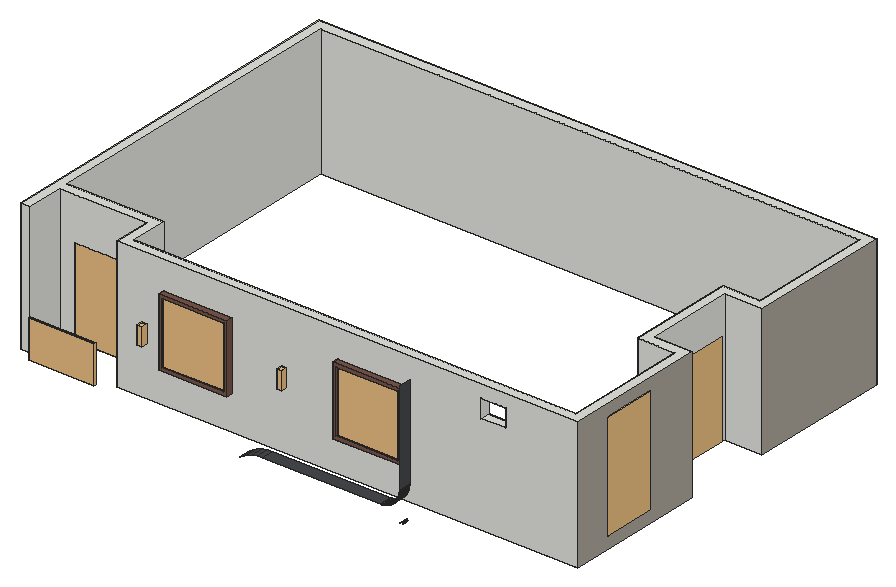
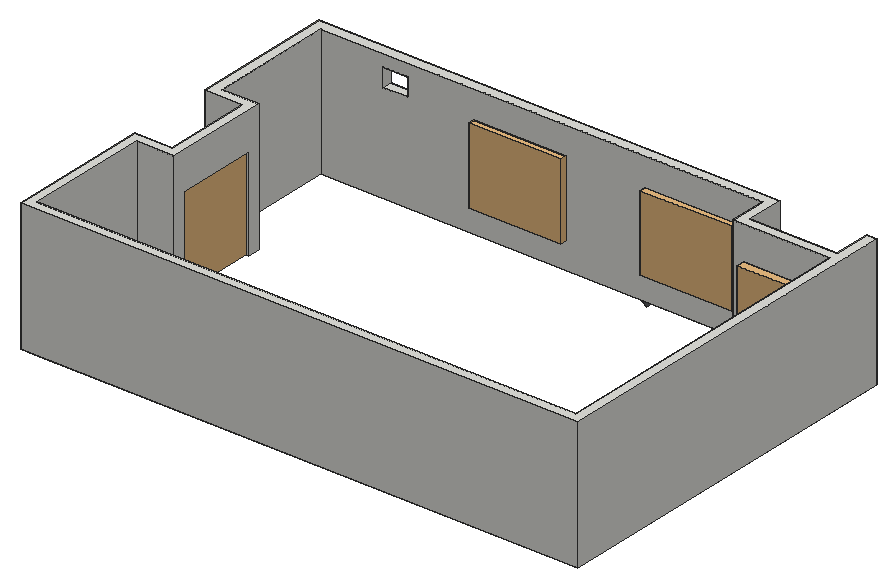
# SketchUp Ruby script. Lengths in inches.
U = 1.inch
M = Sketchup.active_model
def pt(a) = Geom::Point3d.new(a.map { |v| v * U })
def face(e, loops, mat)
  f = e.add_face(loops[0].map { |a| pt(a) })
  loops[1..].each { |l| e.add_face(l.map { |a| pt(a) }).erase! }
  f.material = f.back_material = mat if mat
  f
end
# faces: each face lists its corners as indices into pts; further lists are holes
def faces(e, pts, list, mat = nil) = list.each { |f| face(e, (f[0].is_a?(Array) ? f : [f]).map { |l| l.map { |i| pts[i] } }, mat) }
# xy, xz, yz: faces in a plane at the given z, y or x. An outline is a flat list of corners, or four numbers for a rectangle; further outlines are holes
def ring(l) = l.size == 4 ? [[l[0], l[1]], [l[2], l[1]], [l[2], l[3]], [l[0], l[3]]] : l.each_slice(2).to_a
def flat(e, list, mat, &to3) = list.each { |f| face(e, (f[0].is_a?(Array) ? f : [f]).map { |l| ring(l).map { |u, v| to3.(u, v) } }, mat) }
def xy(e, z, list, mat = nil) = flat(e, list, mat) { |x, y| [x, y, z] }
def xz(e, y, list, mat = nil) = flat(e, list, mat) { |x, z| [x, y, z] }
def yz(e, x, list, mat = nil) = flat(e, list, mat) { |y, z| [x, y, z] }
def lines(e, pts, list) = list.each { |a, b| e.add_line(pt(pts[a]), pt(pts[b])) }
# prism: a flat outline (further loops are holes) pulled along v
def prism(e, loops, v, mat = nil)
  f = face(e, loops, mat); d = Geom::Vector3d.new(v.map { |x| x * U })
  f.pushpull(f.normal.samedirection?(d) ? d.length : -d.length)
end
def box(e, o, s, mat = nil) = prism(e, [[o, [o[0] + s[0], o[1], o[2]], [o[0] + s[0], o[1] + s[1], o[2]], [o[0], o[1] + s[1], o[2]]]], [0, 0, s[2]], mat)
def at(x, y, z, deg = 0) = Geom::Transformation.translation(pt([x, y, z])) * Geom::Transformation.rotation(ORIGIN, Z_AXIS, deg.degrees)
def axes(o, x, y, z) = Geom::Transformation.new([*x, 0, *y, 0, *z, 0, *pt(o).to_a, 1])
def part(name) = M.definitions.add(name)
# library, detail: a bought-in or finely detailed component or shape, given as its bounding box
def library(name, o, s) = part(name).tap { |d| box(d.entities, o, s) }
def detail(e, o, s) = box(e.add_group.entities, o, s)
def put(e, d, t, mat = nil) = e.add_instance(d, t).tap { |i| i.material = mat if mat }
def group(e, t, mat = nil) = e.add_group.tap { |g| g.transformation = t; g.material = mat if mat }.entities
root = M.entities
M.materials.add("1111 AP 9939 Brown seed-N").color = [120, 84, 73]
M.materials.add("1432 AP 8245 TAR ROAD").color = [71, 72, 75]
M.materials.add("Generic").color = [172, 166, 153]
M.materials.add("Outer Light").color = [251, 217, 152]
M.materials.add("[Granite Dark Gray]").color = [69, 68, 68]
M.materials.add("[Wood Cherry Original]").color = [152, 86, 42]
M.materials.add("[Wood Veneer 01]").color = [120, 70, 37]
c1 = library("Group\#43",[0,-2,0],[63,2,36])
c2 = library("WALL LIGHT 69",[4.19,4.05,-8.78],[4.61,5.7,17.13])
c3 = library("Double-hung window 69 in. x 58 in. triple row with mullions",[0,0,-3.59],[62,58,4.59])
c4 = library("Glass Door",[0,0,0],[72,3.54,96])
c5 = library("RIDEAUX \#16",[0,0,0],[103.86,7.74,93.57])
c6 = library("Curtain",[0,0,0],[121.12,7.86,100.24])
c7 = library("SLIDING+GLASS+DOOR",[0,-0.75,0],[72,5.75,80])
c8 = library("Group\#20",[0,0,0],[0.5,51,102])
xy(root,302.79,[[279,95.37,393,107.37],[393,95.37,393.24,107.37]],"1432 AP 8245 TAR ROAD")
yz(root,410.99,[[95.37,320.09,107.37,320.32]],"1432 AP 8245 TAR ROAD")
yz(root,411,[[95.37,320.56,107.37,320.79],[95.37,320.79,107.37,410.79]],"1432 AP 8245 TAR ROAD")
p = [[413.94,96.87,292.75],[414.31,96.87,293.02],[414.31,95.37,293.02],[413.94,95.37,292.75],[411.97,95.37,293.18],[411.61,95.37,292.9375],
  [411.61,96.87,292.9375],[411.97,96.87,293.18],[411.97,96.87,293.18],[411.61,96.87,292.9375],[411.61,95.37,292.9375],[411.97,95.37,293.18],
  [414.67,96.87,293.31],[414.67,95.37,293.31],[414.31,95.37,293.02],[414.67,95.37,293.31],[414.67,96.87,293.31],[414.31,96.87,293.02],
  [412.33,95.37,293.43],[412.33,96.87,293.43],[412.33,96.87,293.43],[412.33,95.37,293.43],[415.03,96.87,293.59],[415.03,95.37,293.59],
  [415.03,95.37,293.59],[415.03,96.87,293.59],[412.69,95.37,293.69],[412.69,96.87,293.69],[412.69,96.87,293.69],[412.69,95.37,293.69],
  [415.38,96.87,293.88],[415.38,95.37,293.88],[415.38,95.37,293.88],[415.38,96.87,293.88],[413.04,95.37,293.95],[413.04,96.87,293.95],
  [413.04,96.87,293.95],[413.04,95.37,293.95],[415.73,96.87,294.18],[415.73,95.37,294.18],[415.73,95.37,294.18],[415.73,96.87,294.18],
  [413.39,95.37,294.21],[413.39,96.87,294.21],[413.39,96.87,294.21],[413.39,95.37,294.21],[413.74,95.37,294.48],[413.74,96.87,294.48],
  [413.74,96.87,294.48],[413.74,95.37,294.48],[416.08,96.87,294.48],[416.08,95.37,294.48],[416.08,95.37,294.48],[416.08,96.87,294.48],
  [414.08,95.37,294.76],[414.08,96.87,294.76],[414.08,96.87,294.76],[414.08,95.37,294.76],[416.42,96.87,294.78],[416.42,95.37,294.78],
  [416.42,95.37,294.78],[416.42,96.87,294.78],[414.42,95.37,295.04],[414.42,96.87,295.04],[414.42,96.87,295.04],[414.42,95.37,295.04],
  [416.76,96.87,295.09],[416.76,95.37,295.09],[416.76,95.37,295.09],[416.76,96.87,295.09],[414.76,95.37,295.32],[414.76,96.87,295.32],
  [414.76,96.87,295.32],[414.76,95.37,295.32],[417.09,96.87,295.4],[417.09,95.37,295.4],[417.09,95.37,295.4],[417.09,96.87,295.4],
  [415.09,95.37,295.61],[415.09,96.87,295.61],[415.09,96.87,295.61],[415.09,95.37,295.61],[261,107.37,297.97],[257.08,107.37,295.35],
  [257.08,95.37,295.35],[261,95.37,297.97],[417.42,96.87,295.72],[417.42,95.37,295.72],[415.42,95.37,295.9],[415.42,96.87,295.9],
  [415.42,96.87,295.9],[415.42,95.37,295.9],[415.74,95.37,296.19],[415.74,96.87,296.19],[415.74,96.87,296.19],[415.74,95.37,296.19],
  [416.06,95.37,296.49],[416.06,96.87,296.49],[416.06,96.87,296.49],[416.06,95.37,296.49],[416.375,95.37,296.8],[416.375,96.87,296.8],
  [416.375,96.87,296.8],[416.375,95.37,296.8],[416.6875,95.37,297.1],[416.6875,96.87,297.1],[416.6875,96.87,297.1],[416.6875,95.37,297.1],
  [417,95.37,297.42],[417,96.87,297.42],[417,96.87,297.42],[417,95.37,297.42],[417.3,95.37,297.73],[417.3,96.87,297.73],
  [417.3,96.87,297.73],[417.3,95.37,297.73],[265.22,107.37,300.05],[265.22,95.37,300.05],[269.68,107.37,301.57],[269.68,95.37,301.57],
  [274.3,107.37,302.48],[274.3,95.37,302.48],[279,107.37,302.79],[279,95.37,302.79],[393.47,107.37,302.8],[393.24,107.37,302.79],
  [393.24,95.37,302.79],[393.47,95.37,302.8],[393.71,107.37,302.81],[393.71,95.37,302.81],[393.94,107.37,302.82],[393.94,95.37,302.82],
  [394.18,107.37,302.83],[394.18,95.37,302.83],[394.41,107.37,302.85],[394.41,95.37,302.85],[394.65,107.37,302.87],[394.65,95.37,302.87],
  [394.88,107.37,302.89],[394.88,95.37,302.89],[395.12,107.37,302.92],[395.12,95.37,302.92],[395.35,107.37,302.95],[395.35,95.37,302.95],
  [395.58,107.37,302.98],[395.58,95.37,302.98],[395.82,107.37,303.01],[395.82,95.37,303.01],[396.05,107.37,303.05],[396.05,95.37,303.05],
  [396.28,107.37,303.09],[396.28,95.37,303.09],[396.51,107.37,303.14],[396.51,95.37,303.14],[396.74,107.37,303.19],[396.74,95.37,303.19],
  [396.97,107.37,303.24],[396.97,95.37,303.24],[397.2,107.37,303.29],[397.2,95.37,303.29],[397.43,107.37,303.35],[397.43,95.37,303.35],
  [397.66,107.37,303.41],[397.66,95.37,303.41],[397.89,107.37,303.47],[397.89,95.37,303.47],[398.11,107.37,303.53],[398.11,95.37,303.53],
  [398.34,107.37,303.6],[398.34,95.37,303.6],[398.5625,107.37,303.67],[398.5625,95.37,303.67],[398.79,107.37,303.75],[398.79,95.37,303.75],
  [399.01,107.37,303.82],[399.01,95.37,303.82],[399.23,107.37,303.9],[399.23,95.37,303.9],[399.45,107.37,303.99],[399.45,95.37,303.99],
  [399.67,107.37,304.07],[399.67,95.37,304.07],[399.89,107.37,304.16],[399.89,95.37,304.16],[400.11,107.37,304.25],[400.11,95.37,304.25],
  [400.32,107.37,304.35],[400.32,95.37,304.35],[400.54,107.37,304.45],[400.54,95.37,304.45],[400.75,107.37,304.55],[400.75,95.37,304.55],
  [400.96,107.37,304.65],[400.96,95.37,304.65],[401.17,107.37,304.75],[401.17,95.37,304.75],[401.38,107.37,304.86],[401.38,95.37,304.86],
  [401.59,107.37,304.97],[401.59,95.37,304.97],[401.8,107.37,305.09],[401.8,95.37,305.09],[402,107.37,305.2],[402,95.37,305.2],
  [402.2,107.37,305.32],[402.2,95.37,305.32],[402.4,107.37,305.44],[402.4,95.37,305.44],[402.61,107.37,305.57],[402.61,95.37,305.57],
  [402.8,107.37,305.7],[402.8,95.37,305.7],[403,107.37,305.83],[403,95.37,305.83],[403.2,107.37,305.96],[403.2,95.37,305.96],
  [403.39,107.37,306.09],[403.39,95.37,306.09],[403.58,107.37,306.23],[403.58,95.37,306.23],[403.77,107.37,306.37],[403.77,95.37,306.37],
  [403.96,107.37,306.51],[403.96,95.37,306.51],[404.14,107.37,306.66],[404.14,95.37,306.66],[404.33,107.37,306.8],[404.33,95.37,306.8],
  [404.51,107.37,306.95],[404.51,95.37,306.95],[404.69,107.37,307.1],[404.69,95.37,307.1],[404.87,107.37,307.26],[404.87,95.37,307.26],
  [405.04,107.37,307.42],[405.04,95.37,307.42],[405.22,107.37,307.57],[405.22,95.37,307.57],[405.39,107.37,307.74],[405.39,95.37,307.74],
  [405.56,107.37,307.9],[405.56,95.37,307.9],[405.73,107.37,308.0625],[405.73,95.37,308.0625],[405.89,107.37,308.23],[405.89,95.37,308.23],
  [406.06,107.37,308.4],[406.06,95.37,308.4],[406.22,107.37,308.57],[406.22,95.37,308.57],[406.375,107.37,308.75],[406.375,95.37,308.75],
  [406.53,107.37,308.92],[406.53,95.37,308.92],[406.6875,107.37,309.1],[406.6875,95.37,309.1],[406.84,107.37,309.28],[406.84,95.37,309.28],
  [406.99,107.37,309.46],[406.99,95.37,309.46],[407.14,107.37,309.65],[407.14,95.37,309.65],[407.28,107.37,309.83],[407.28,95.37,309.83],
  [407.42,107.37,310.02],[407.42,95.37,310.02],[407.5625,107.37,310.21],[407.5625,95.37,310.21],[407.7,107.37,310.4],[407.7,95.37,310.4],
  [407.83,107.37,310.6],[407.83,95.37,310.6],[407.97,107.37,310.79],[407.97,95.37,310.79],[408.1,107.37,310.99],[408.1,95.37,310.99],
  [408.22,107.37,311.1875],[408.22,95.37,311.1875],[408.35,107.37,311.39],[408.35,95.37,311.39],[408.47,107.37,311.59],[408.47,95.37,311.59],
  [408.59,107.37,311.79],[408.59,95.37,311.79],[408.7,107.37,312],[408.7,95.37,312],[408.82,107.37,312.2],[408.82,95.37,312.2],
  [408.93,107.37,312.41],[408.93,95.37,312.41],[409.04,107.37,312.62],[409.04,95.37,312.62],[409.14,107.37,312.83],[409.14,95.37,312.83],
  [409.25,107.37,313.04],[409.25,95.37,313.04],[409.35,107.37,313.26],[409.35,95.37,313.26],[409.44,107.37,313.47],[409.44,95.37,313.47],
  [409.54,107.37,313.6875],[409.54,95.37,313.6875],[409.63,107.37,313.9],[409.63,95.37,313.9],[409.72,107.37,314.12],[409.72,95.37,314.12],
  [409.8,107.37,314.34],[409.8,95.37,314.34],[409.89,107.37,314.5625],[409.89,95.37,314.5625],[409.97,107.37,314.78],[409.97,95.37,314.78],
  [410.04,107.37,315.01],[410.04,95.37,315.01],[410.12,107.37,315.23],[410.12,95.37,315.23],[410.19,107.37,315.45],[410.19,95.37,315.45],
  [410.26,107.37,315.68],[410.26,95.37,315.68],[410.32,107.37,315.91],[410.32,95.37,315.91],[410.39,107.37,316.13],[410.39,95.37,316.13],
  [410.45,107.37,316.36],[410.45,95.37,316.36],[410.5,107.37,316.59],[410.5,95.37,316.59],[410.56,107.37,316.82],[410.56,95.37,316.82],
  [410.61,107.37,317.05],[410.61,95.37,317.05],[410.65,107.37,317.28],[410.65,95.37,317.28],[410.7,107.37,317.51],[410.7,95.37,317.51],
  [410.74,107.37,317.74],[410.74,95.37,317.74],[410.78,107.37,317.98],[410.78,95.37,317.98],[410.8125,107.37,318.21],[410.8125,95.37,318.21],
  [410.85,107.37,318.44],[410.85,95.37,318.44],[410.875,107.37,318.68],[410.875,95.37,318.68],[410.9,107.37,318.91],[410.9,95.37,318.91],
  [410.92,107.37,319.15],[410.92,95.37,319.15],[410.94,107.37,319.38],[410.94,95.37,319.38],[410.96,107.37,319.61],[410.96,95.37,319.61],
  [410.98,107.37,319.85],[410.98,95.37,319.85],[410.99,107.37,320.09],[410.99,95.37,320.09],[411,107.37,320.56],[410.99,107.37,320.32],
  [410.99,95.37,320.32],[411,95.37,320.56]]
faces(root,p,[[0,1,2,3],[8,9,10,11],[1,12,13,2],[20,8,11,21],[12,22,23,13],[28,20,21,29],[22,30,31,23],[36,28,29,37],
  [30,38,39,31],[44,36,37,45],[48,44,45,49],[38,50,51,39],[56,48,49,57],[50,58,59,51],[64,56,57,65],[58,66,67,59],
  [72,64,65,73],[66,74,75,67],[80,72,73,81],[74,86,87,75],[90,80,81,91],[94,90,91,95],[98,94,95,99],[102,98,99,103],
  [106,102,103,107],[110,106,107,111],[114,110,111,115]],"Outer Light")
faces(root,p,[[4,5,6,7],[14,15,16,17],[18,4,7,19],[15,24,25,16],[26,18,19,27],[24,32,33,25],[34,26,27,35],[32,40,41,33],
  [42,34,35,43],[46,42,43,47],[40,52,53,41],[54,46,47,55],[52,60,61,53],[62,54,55,63],[60,68,69,61],[70,62,63,71],
  [68,76,77,69],[78,70,71,79],[82,83,84,85],[88,78,79,89],[92,88,89,93],[96,92,93,97],[100,96,97,101],[104,100,101,105],
  [108,104,105,109],[112,108,109,113],[116,82,85,117],[118,116,117,119],[120,118,119,121],[122,120,121,123],[124,125,126,127],[128,124,127,129],
  [130,128,129,131],[132,130,131,133],[134,132,133,135],[136,134,135,137],[138,136,137,139],[140,138,139,141],[142,140,141,143],[144,142,143,145],
  [146,144,145,147],[148,146,147,149],[150,148,149,151],[152,150,151,153],[154,152,153,155],[156,154,155,157],[158,156,157,159],[160,158,159,161],
  [162,160,161,163],[164,162,163,165],[166,164,165,167],[168,166,167,169],[170,168,169,171],[172,170,171,173],[174,172,173,175],[176,174,175,177],
  [178,176,177,179],[180,178,179,181],[182,180,181,183],[184,182,183,185],[186,184,185,187],[188,186,187,189],[190,188,189,191],[192,190,191,193],
  [194,192,193,195],[196,194,195,197],[198,196,197,199],[200,198,199,201],[202,200,201,203],[204,202,203,205],[206,204,205,207],[208,206,207,209],
  [210,208,209,211],[212,210,211,213],[214,212,213,215],[216,214,215,217],[218,216,217,219],[220,218,219,221],[222,220,221,223],[224,222,223,225],
  [226,224,225,227],[228,226,227,229],[230,228,229,231],[232,230,231,233],[234,232,233,235],[236,234,235,237],[238,236,237,239],[240,238,239,241],
  [242,240,241,243],[244,242,243,245],[246,244,245,247],[248,246,247,249],[250,248,249,251],[252,250,251,253],[254,252,253,255],[256,254,255,257],
  [258,256,257,259],[260,258,259,261],[262,260,261,263],[264,262,263,265],[266,264,265,267],[268,266,267,269],[270,268,269,271],[272,270,271,273],
  [274,272,273,275],[276,274,275,277],[278,276,277,279],[280,278,279,281],[282,280,281,283],[284,282,283,285],[286,284,285,287],[288,286,287,289],
  [290,288,289,291],[292,290,291,293],[294,292,293,295],[296,294,295,297],[298,296,297,299],[300,298,299,301],[302,300,301,303],[304,302,303,305],
  [306,304,305,307],[308,306,307,309],[310,308,309,311],[312,310,311,313],[314,312,313,315],[316,314,315,317],[318,316,317,319],[320,318,319,321],
  [322,320,321,323],[324,322,323,325],[326,324,325,327],[328,326,327,329],[330,328,329,331],[332,330,331,333],[334,332,333,335],[336,334,335,337],
  [338,336,337,339],[340,338,339,341],[342,340,341,343],[344,342,343,345],[346,344,345,347],[348,346,347,349],[350,348,349,351],[352,350,351,353],
  [354,352,353,355],[356,354,355,357],[358,359,360,361]],"1432 AP 8245 TAR ROAD")
put(root,c1,at(51,100.37,305.79),"[Wood Cherry Original]")
put(root,c2,at(148.76,97.62,361.66))
put(root,c2,at(283.52,97.62,371.25))
g1 = group(root,at(36,101.37,308.79))
xy(g1,-3,[[0,6,0,366,528,366,528,357,9,357,9,51,24,51,24,42,9,42,9,6],[93,6,93,42,78,42,78,51,102,51,102,15,528,15,528,135,492,135,492,147,501,147,501,144,537,144,537,6],[492,225,492,237,528,237,528,366,537,366,537,228,501,228,501,225]])
xy(g1,30,[[138,0,204,6],[306,0,372,6]],"1111 AP 9939 Brown seed-N")
xy(g1,33,[[141,0,201,15],[309,0,369,15]],"1111 AP 9939 Brown seed-N")
xy(g1,81,[[24,42,78,51]])
xy(g1,87,[[492,147,501,225]])
xy(g1,93,[[444,6,468,15]])
xy(g1,93,[[141,0,201,15],[309,0,369,15]],"1111 AP 9939 Brown seed-N")
xy(g1,96,[[138,0,204,6],[306,0,372,6]],"1111 AP 9939 Brown seed-N")
xy(g1,111,[[444,6,468,15]])
xy(g1,123,[[[0,6,9,6,9,42,93,42,93,6,537,6,537,144,501,144,501,228,537,228,537,366,0,366],[102,15,102,51,9,51,9,357,528,357,528,237,492,237,492,135,528,135,528,15]]])
xz(g1,0,[[[138,30,204,96],[141,33,201,93]],[[306,30,372,96],[309,33,369,93]]],"1111 AP 9939 Brown seed-N")
xz(g1,6,[[0,-3,9,123],[[93,-3,537,123],[138,30,204,96],[306,30,372,96],[444,93,468,111]]])
xz(g1,15,[[[102,-3,528,123],[309,33,369,93],[141,33,201,93],[444,93,468,111]]])
xz(g1,42,[[9,-3,24,-3,24,81,78,81,78,-3,93,-3,93,123,9,123]])
xz(g1,51,[[9,-3,9,123,102,123,102,-3,78,-3,78,81,24,81,24,-3]])
xz(g1,135,[[492,-3,528,123]])
xz(g1,144,[[501,-3,537,123]])
xz(g1,147,[[492,-3,501,87]])
xz(g1,225,[[492,-3,501,87]])
xz(g1,228,[[501,-3,537,123]])
xz(g1,237,[[492,-3,528,123]])
xz(g1,357,[[9,-3,528,123]])
xz(g1,366,[[0,-3,537,123]])
yz(g1,0,[[6,-3,366,123]])
yz(g1,9,[[6,-3,42,123],[51,-3,357,123]])
yz(g1,24,[[42,-3,51,81]])
yz(g1,78,[[42,-3,51,81]])
yz(g1,93,[[6,-3,42,123]])
yz(g1,102,[[15,-3,51,123]])
yz(g1,138,[[0,30,6,96]],"1111 AP 9939 Brown seed-N")
yz(g1,141,[[0,33,15,93]],"1111 AP 9939 Brown seed-N")
yz(g1,201,[[0,33,15,93]],"1111 AP 9939 Brown seed-N")
yz(g1,204,[[0,30,6,96]],"1111 AP 9939 Brown seed-N")
yz(g1,306,[[0,30,6,96]],"1111 AP 9939 Brown seed-N")
yz(g1,309,[[0,33,15,93]],"1111 AP 9939 Brown seed-N")
yz(g1,369,[[0,33,15,93]],"1111 AP 9939 Brown seed-N")
yz(g1,372,[[0,30,6,96]])
yz(g1,444,[[6,93,15,111]])
yz(g1,468,[[6,93,15,111]])
yz(g1,492,[[135,-3,135,123,237,123,237,-3,225,-3,225,87,147,87,147,-3]])
yz(g1,501,[[144,-3,147,-3,147,87,225,87,225,-3,228,-3,228,123,144,123]])
yz(g1,528,[[15,-3,135,123],[237,-3,357,123]])
yz(g1,537,[[59.76,9,93,9,93,111,59.76,111,59.53,110.99,59.29,110.99,59.06,110.98,58.82,110.96,58.59,110.94,58.35,110.92,58.12,110.9,57.88,110.875,57.65,110.85,57.42,110.8125,57.18,110.78,56.72,110.7,56.49,110.65,56.26,110.61,56.03,110.56,55.8,110.5,55.57,110.45,55.34,110.39,55.11,110.32,54.89,110.26,54.66,110.19,54.4375,110.12,54.21,110.04,53.99,109.97,53.77,109.89,53.55,109.8,53.33,109.72,52.89,109.54,52.68,109.44,52.46,109.35,52.25,109.25,52.04,109.14,51.83,109.04,51.41,108.82,51.2,108.7,51,108.59,50.6,108.35,50.39,108.22,50.2,108.1,50,107.97,49.8,107.83,49.61,107.7,49.42,107.5625,49.23,107.42,49.04,107.28,48.86,107.14,48.67,106.99,48.49,106.84,48.31,106.6875,48.13,106.53,47.96,106.375,47.78,106.22,47.61,106.06,47.44,105.89,47.27,105.73,47.11,105.56,46.94,105.39,46.78,105.22,46.625,105.04,46.47,104.87,46.3125,104.69,46.16,104.51,46.01,104.33,45.86,104.14,45.72,103.96,45.58,103.77,45.4375,103.58,45.3,103.39,45.17,103.2,45.03,103,44.9,102.8,44.78,102.61,44.65,102.4,44.41,102,44.3,101.8,44.18,101.59,43.96,101.17,43.86,100.96,43.75,100.75,43.65,100.54,43.56,100.32,43.46,100.11,43.28,99.67,43.2,99.45,43.11,99.23,43.03,99.01,42.96,98.79,42.88,98.5625,42.81,98.34,42.74,98.11,42.68,97.89,42.61,97.66,42.55,97.43,42.5,97.2,42.44,96.97,42.39,96.74,42.35,96.51,42.3,96.28,42.22,95.82,42.1875,95.58,42.15,95.35,42.125,95.12,42.1,94.88,42.08,94.65,42.06,94.41,42.04,94.18,42.02,93.94,42.01,93.71,42.01,93.47,42,93.24,42,26.76,42.01,26.53,42.01,26.29,42.02,26.06,42.04,25.82,42.06,25.59,42.08,25.35,42.1,25.12,42.125,24.88,42.15,24.65,42.1875,24.42,42.22,24.18,42.3,23.72,42.35,23.49,42.39,23.26,42.44,23.03,42.5,22.8,42.55,22.57,42.61,22.34,42.68,22.11,42.74,21.89,42.81,21.66,42.88,21.4375,42.96,21.21,43.03,20.99,43.11,20.77,43.2,20.55,43.28,20.33,43.46,19.89,43.56,19.68,43.65,19.46,43.75,19.25,43.86,19.04,43.96,18.83,44.18,18.41,44.3,18.2,44.41,18,44.65,17.6,44.78,17.39,44.9,17.2,45.03,17,45.17,16.8,45.3,16.61,45.4375,16.42,45.58,16.23,45.72,16.04,45.86,15.86,46.01,15.67,46.16,15.49,46.3125,15.31,46.47,15.13,46.625,14.96,46.78,14.78,46.94,14.61,47.11,14.44,47.27,14.27,47.44,14.11,47.61,13.94,47.78,13.78,47.96,13.625,48.13,13.47,48.31,13.3125,48.49,13.16,48.67,13.01,48.86,12.86,49.04,12.72,49.23,12.58,49.42,12.4375,49.61,12.3,49.8,12.17,50,12.03,50.2,11.9,50.39,11.78,50.6,11.65,51,11.41,51.2,11.3,51.41,11.18,51.83,10.96,52.04,10.86,52.25,10.75,52.46,10.65,52.68,10.56,52.89,10.46,53.33,10.28,53.55,10.2,53.77,10.11,53.99,10.03,54.21,9.96,54.4375,9.88,54.66,9.81,54.89,9.74,55.11,9.68,55.34,9.61,55.57,9.55,55.8,9.5,56.03,9.44,56.26,9.39,56.49,9.35,56.72,9.3,57.18,9.22,57.42,9.1875,57.65,9.15,57.88,9.125,58.12,9.1,58.35,9.08,58.59,9.06,58.82,9.04,59.06,9.02,59.29,9.01,59.53,9.01]])
yz(g1,537,[[[6,-3,144,123],[59.76,9,59.53,9.01,59.29,9.01,59.06,9.02,58.82,9.04,58.59,9.06,58.35,9.08,58.12,9.1,57.88,9.125,57.65,9.15,57.42,9.1875,57.18,9.22,56.72,9.3,56.49,9.35,56.26,9.39,56.03,9.44,55.8,9.5,55.57,9.55,55.34,9.61,55.11,9.68,54.89,9.74,54.66,9.81,54.4375,9.88,54.21,9.96,53.99,10.03,53.77,10.11,53.55,10.2,53.33,10.28,52.89,10.46,52.68,10.56,52.46,10.65,52.25,10.75,52.04,10.86,51.83,10.96,51.41,11.18,51.2,11.3,51,11.41,50.6,11.65,50.39,11.78,50.2,11.9,50,12.03,49.8,12.17,49.61,12.3,49.42,12.4375,49.23,12.58,49.04,12.72,48.86,12.86,48.67,13.01,48.49,13.16,48.31,13.3125,48.13,13.47,47.96,13.625,47.78,13.78,47.61,13.94,47.44,14.11,47.27,14.27,47.11,14.44,46.94,14.61,46.78,14.78,46.625,14.96,46.47,15.13,46.3125,15.31,46.16,15.49,46.01,15.67,45.86,15.86,45.72,16.04,45.58,16.23,45.4375,16.42,45.3,16.61,45.17,16.8,45.03,17,44.9,17.2,44.78,17.39,44.65,17.6,44.41,18,44.3,18.2,44.18,18.41,43.96,18.83,43.86,19.04,43.75,19.25,43.65,19.46,43.56,19.68,43.46,19.89,43.28,20.33,43.2,20.55,43.11,20.77,43.03,20.99,42.96,21.21,42.88,21.4375,42.81,21.66,42.74,21.89,42.68,22.11,42.61,22.34,42.55,22.57,42.5,22.8,42.44,23.03,42.39,23.26,42.35,23.49,42.3,23.72,42.22,24.18,42.1875,24.42,42.15,24.65,42.125,24.88,42.1,25.12,42.08,25.35,42.06,25.59,42.04,25.82,42.02,26.06,42.01,26.29,42.01,26.53,42,26.76,42,93.24,42.01,93.47,42.01,93.71,42.02,93.94,42.04,94.18,42.06,94.41,42.08,94.65,42.1,94.88,42.125,95.12,42.15,95.35,42.1875,95.58,42.22,95.82,42.3,96.28,42.35,96.51,42.39,96.74,42.44,96.97,42.5,97.2,42.55,97.43,42.61,97.66,42.68,97.89,42.74,98.11,42.81,98.34,42.88,98.5625,42.96,98.79,43.03,99.01,43.11,99.23,43.2,99.45,43.28,99.67,43.46,100.11,43.56,100.32,43.65,100.54,43.75,100.75,43.86,100.96,43.96,101.17,44.18,101.59,44.3,101.8,44.41,102,44.65,102.4,44.78,102.61,44.9,102.8,45.03,103,45.17,103.2,45.3,103.39,45.4375,103.58,45.58,103.77,45.72,103.96,45.86,104.14,46.01,104.33,46.16,104.51,46.3125,104.69,46.47,104.87,46.625,105.04,46.78,105.22,46.94,105.39,47.11,105.56,47.27,105.73,47.44,105.89,47.61,106.06,47.78,106.22,47.96,106.375,48.13,106.53,48.31,106.6875,48.49,106.84,48.67,106.99,48.86,107.14,49.04,107.28,49.23,107.42,49.42,107.5625,49.61,107.7,49.8,107.83,50,107.97,50.2,108.1,50.39,108.22,50.6,108.35,51,108.59,51.2,108.7,51.41,108.82,51.83,109.04,52.04,109.14,52.25,109.25,52.46,109.35,52.68,109.44,52.89,109.54,53.33,109.72,53.55,109.8,53.77,109.89,53.99,109.97,54.21,110.04,54.4375,110.12,54.66,110.19,54.89,110.26,55.11,110.32,55.34,110.39,55.57,110.45,55.8,110.5,56.03,110.56,56.26,110.61,56.49,110.65,56.72,110.7,57.18,110.78,57.42,110.8125,57.65,110.85,57.88,110.875,58.12,110.9,58.35,110.92,58.59,110.94,58.82,110.96,59.06,110.98,59.29,110.99,59.53,110.99,59.76,111,93,111,93,9]],[228,-3,366,123]],"Generic")
put(g1,c3,axes([201,4.5,33],[-0.96774,0,0],[0,0,1.03448],[0,0.696,0]),"[Granite Dark Gray]")
put(g1,c3,axes([369,4.5,33],[-0.96774,0,0],[0,0,1.03448],[0,0.696,0]),"[Granite Dark Gray]")
put(g1,c4,axes([24,42,-3],[0.75,0,0],[0,0.74,0],[0,0,0.875]))
put(g1,c5,axes([9,51,-3],[0.79912,0,0],[0,1,0],[0,0,1]))
put(g1,c6,axes([127.26,15,22.18],[0.73,0,0],[0,0.73,0],[0,0,0.73]))
put(g1,c6,axes([292.51,15,22.18],[0.73,0,0],[0,0.73,0],[0,0,0.73]))
put(g1,c7,axes([496,225,-3],[0,-1.08333,0],[1,0,0],[0,0,1.125]))
put(g1,c8,at(537,42,9),"[Wood Veneer 01]")
